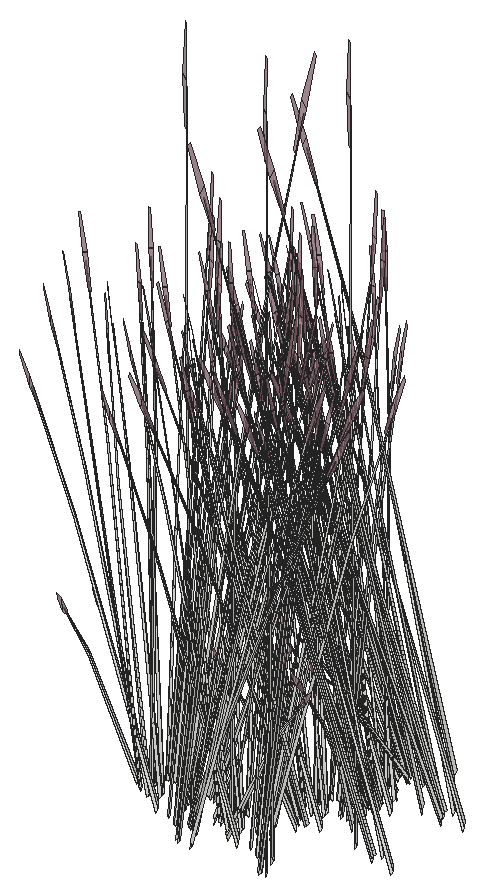
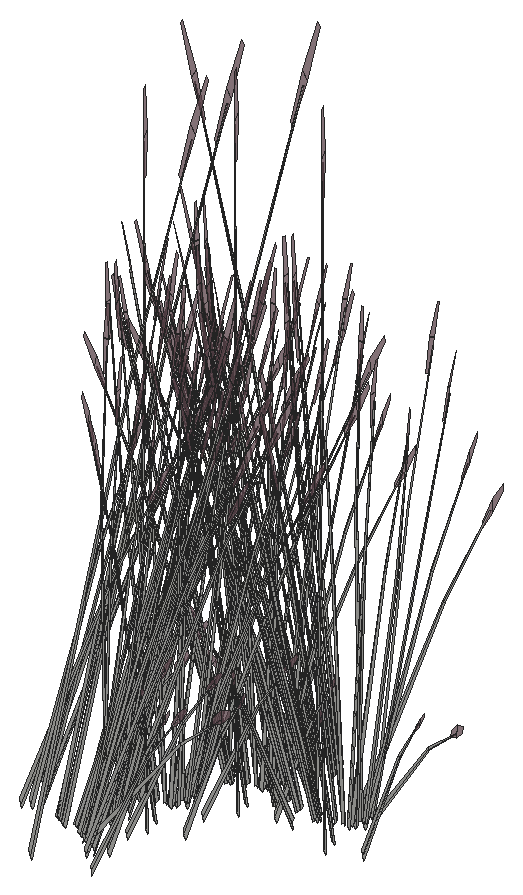
# SketchUp Ruby script. Lengths in inches.
U = 1.inch
M = Sketchup.active_model
def pt(a) = Geom::Point3d.new(a.map { |v| v * U })
def face(e, loops, mat)
  f = e.add_face(loops[0].map { |a| pt(a) })
  loops[1..].each { |l| e.add_face(l.map { |a| pt(a) }).erase! }
  f.material = f.back_material = mat if mat
  f
end
# faces: each face lists its corners as indices into pts; further lists are holes
def faces(e, pts, list, mat = nil) = list.each { |f| face(e, (f[0].is_a?(Array) ? f : [f]).map { |l| l.map { |i| pts[i] } }, mat) }
# xy, xz, yz: faces in a plane at the given z, y or x. An outline is a flat list of corners, or four numbers for a rectangle; further outlines are holes
def ring(l) = l.size == 4 ? [[l[0], l[1]], [l[2], l[1]], [l[2], l[3]], [l[0], l[3]]] : l.each_slice(2).to_a
def flat(e, list, mat, &to3) = list.each { |f| face(e, (f[0].is_a?(Array) ? f : [f]).map { |l| ring(l).map { |u, v| to3.(u, v) } }, mat) }
def xy(e, z, list, mat = nil) = flat(e, list, mat) { |x, y| [x, y, z] }
def xz(e, y, list, mat = nil) = flat(e, list, mat) { |x, z| [x, y, z] }
def yz(e, x, list, mat = nil) = flat(e, list, mat) { |y, z| [x, y, z] }
def lines(e, pts, list) = list.each { |a, b| e.add_line(pt(pts[a]), pt(pts[b])) }
# prism: a flat outline (further loops are holes) pulled along v
def prism(e, loops, v, mat = nil)
  f = face(e, loops, mat); d = Geom::Vector3d.new(v.map { |x| x * U })
  f.pushpull(f.normal.samedirection?(d) ? d.length : -d.length)
end
def box(e, o, s, mat = nil) = prism(e, [[o, [o[0] + s[0], o[1], o[2]], [o[0] + s[0], o[1] + s[1], o[2]], [o[0], o[1] + s[1], o[2]]]], [0, 0, s[2]], mat)
def at(x, y, z, deg = 0) = Geom::Transformation.translation(pt([x, y, z])) * Geom::Transformation.rotation(ORIGIN, Z_AXIS, deg.degrees)
def axes(o, x, y, z) = Geom::Transformation.new([*x, 0, *y, 0, *z, 0, *pt(o).to_a, 1])
def part(name) = M.definitions.add(name)
# library, detail: a bought-in or finely detailed component or shape, given as its bounding box
def library(name, o, s) = part(name).tap { |d| box(d.entities, o, s) }
def detail(e, o, s) = box(e.add_group.entities, o, s)
def put(e, d, t, mat = nil) = e.add_instance(d, t).tap { |i| i.material = mat if mat }
def group(e, t, mat = nil) = e.add_group.tap { |g| g.transformation = t; g.material = mat if mat }.entities
root = M.entities
M.materials.add("LightPink_Translucent").color = [144, 107, 117]
M.materials["LightPink_Translucent"].alpha = 0.75
c1 = part("blade")
p = [[2.15,0.21,22],[0,0.17,0],[0.09,0.45,0],[2.18,0.31,22],[2.29,0.31,22],[0.38,0.45,0],
  [2.48,0.24,33],[2.49,0.24,33],[2.48,0.22,33]]
faces(c1.entities,p,[[0,1,2,3],[4,5,2,3],[6,3,4,7],[8,0,3,6]])
c2 = part("seeds")
p = [[0.3,-0.1,1.38],[-0.01,-0.03,1.59],[-0.01,-0.03,0.03],[0.14,-0.07,-0.07],[0.29,-0.03,3],[0.15,0.01,3.11]]
faces(c2.entities,p,[[0,1,2,3],[1,0,4,5]],"LightPink_Translucent")
c3 = part("blade with seeds")
put(c3.entities,c1,at(0,0,0))
put(c3.entities,c2,axes([2.4,0.25,30.99],[1.5799,-0.05474,1.17369],[-0.12525,1.92788,0.29478],[-0.07173,-0.02425,1.56792]))
put(root,c3,axes([332.89,18.93,50.44],[-0.01307,-0.23234,1.01491],[0.32652,0.16572,0.74569],[-0.06422,0.11074,0.22354]))
put(root,c3,axes([326.85,20.29,51.43],[-0.20943,0.00885,1.51428],[0.13893,-0.38357,0.12244],[0.29846,0.02372,0.64734]))
put(root,c3,axes([330.16,19.82,50.95],[0.14352,-0.05653,1.56454],[0.04949,0.39467,0.12244],[-0.31087,0.05237,0.55918]))
put(root,c3,axes([327.35,18.03,52.42],[0.36145,0.26255,-0.50118],[-0.38183,0.22994,-0.3882],[-0.055,0.1334,0.95895]))
put(root,c3,axes([333.01,18.03,52.42],[0.36145,0.26255,-0.50118],[-0.38183,0.22994,-0.3882],[-0.055,0.1334,0.95895]))
put(root,c3,axes([328.43,18.29,52.14],[0.49634,0.09796,-0.45151],[-0.17013,0.33585,-0.34973],[0.04551,0.13522,0.86392]))
put(root,c3,axes([328.71,17.59,51.43],[-0.11542,-0.12546,1.51428],[0.53333,-0.10562,0.12244],[0.12054,0.19696,0.64734]))
put(root,c3,axes([331.92,23.125,51.43],[0.18755,0.06732,1.51428],[-0.38813,0.28243,0.12244],[-0.24191,-0.12741,0.64734]))
put(root,c3,axes([324.34,20.13,50.95],[0.14352,-0.05653,1.56454],[0.04949,0.39467,0.12244],[-0.31087,0.05237,0.55918]))
put(root,c3,axes([328.2,18.49,52],[-0.15222,0.30049,-0.31292],[-0.44409,-0.08764,0.40398],[0.04072,0.12098,0.77298]))
put(root,c3,axes([329.17,20.04,52.14],[-0.13679,0.35544,-0.45151],[-0.46898,-0.12183,-0.34973],[-0.18882,0.03259,0.86392]))
put(root,c3,axes([328.89,20.75,50.44],[-0.31197,0.06451,1.01491],[0.14684,-0.26661,0.74569],[0.1655,0.01824,0.22354]))
put(root,c3,axes([329.15,19.73,52.45],[0.25405,0.35383,-0.10745],[-0.45089,0.17388,-0.59638],[-0.19001,0.04668,0.90619]))
put(root,c3,axes([332.83,22.93,52.14],[-0.49824,0.09289,-0.45151],[-0.08716,-0.35177,-0.34973],[-0.13382,-0.10081,0.86392]))
put(root,c3,axes([327.24,17.91,52.72],[-0.01314,0.36145,-0.69681],[-0.55324,-0.02428,0.08409],[-0.05838,0.15313,0.9857]))
put(root,c3,axes([332.9,17.91,52.72],[-0.01314,0.36145,-0.69681],[-0.55324,-0.02428,0.08409],[-0.05838,0.15313,0.9857]))
put(root,c3,axes([338.15,22.06,52.4],[-0.50473,-0.00941,-0.62776],[0.0339,-0.39618,0.07576],[-0.21383,-0.04181,0.88802]))
put(root,c3,axes([327.76,17.66,51.43],[-0.01236,-0.14998,1.51428],[0.53562,0.09949,0.12244],[-0.03313,0.21373,0.64734]))
put(root,c3,axes([333.42,17.66,51.43],[-0.01236,-0.14998,1.51428],[0.53562,0.09949,0.12244],[-0.03313,0.21373,0.64734]))
put(root,c3,axes([322.8,20.39,52.17],[-0.08245,0.05073,1.54581],[0.00701,0.37067,-0.24447],[-0.18899,0.0482,0.12397]))
put(root,c3,axes([323.35,20.34,52.14],[-0.13679,0.35544,-0.45151],[-0.46898,-0.12183,-0.34973],[-0.18882,0.03259,0.86392]))
put(root,c3,axes([323.33,20.04,52.45],[0.25405,0.35383,-0.10745],[-0.45089,0.17388,-0.59638],[-0.19001,0.04668,0.90619]))
put(root,c3,axes([328.35,21.58,51.47],[-0.09664,-0.32847,-0.03085],[0.45676,-0.07551,-0.13989],[0.09538,0.02082,0.4614]))
put(root,c3,axes([327.16,21.57,52.45],[0.02704,-0.39739,-0.10745],[0.51189,0.01086,-0.59638],[0.19715,0.0276,0.90619]))
put(root,c3,axes([328.25,18.22,52.4],[0.24099,0.31773,-0.62776],[-0.49607,0.17707,0.07576],[0.05635,0.15352,0.88802]))
put(root,c3,axes([334.06,25.06,50.9375],[0.43633,0.15757,1.33654],[-0.42745,0.33945,0.52853],[-0.19146,-0.20119,1.12046]))
put(root,c3,axes([329.15,20.22,51.43],[0.17519,-0.08265,1.51428],[0.14749,0.38193,0.12244],[-0.27504,0.08632,0.64734]))
put(root,c3,axes([327.06,18.42,50.97],[0.01109,-0.20172,1.3638],[0.49896,0.10655,0.18846],[-0.04323,0.21498,0.64398]))
put(root,c3,axes([332.71,18.42,50.97],[0.01109,-0.20172,1.3638],[0.49896,0.10655,0.18846],[-0.04323,0.21498,0.64398]))
put(root,c3,axes([323.34,20.53,51.43],[0.17519,-0.08265,1.51428],[0.14749,0.38193,0.12244],[-0.27504,0.08632,0.64734]))
put(root,c3,axes([337.52,22.42,51.43],[0.20943,-0.00885,1.51428],[-0.13893,0.38357,0.12244],[-0.29846,-0.02372,0.64734]))
put(root,c3,axes([331.85,23.22,52],[-0.28729,-0.24465,-0.31292],[0.32804,-0.23159,0.40398],[-0.16667,-0.03524,0.77298]))
put(root,c3,axes([327.1875,21.375,52.4],[0.50473,0.00941,-0.62776],[-0.0339,0.39618,0.07576],[0.21383,0.04181,0.88802]))
put(root,c3,axes([328.24,21.56,50.44],[0.21042,-0.1771,1.01491],[0.08303,0.28036,0.74569],[-0.15207,0.0502,0.22354]))
put(root,c3,axes([329.04,20.79,52],[-0.43951,0.05584,-0.31292],[-0.11606,-0.31924,0.40398],[-0.12595,0.08575,0.77298]))
put(root,c3,axes([332.15,23.39,52.4],[-0.50473,-0.00941,-0.62776],[0.0339,-0.39618,0.07576],[-0.21383,-0.04181,0.88802]))
put(root,c3,axes([322.43,21.86,50.44],[0.21042,-0.1771,1.01491],[0.08303,0.28036,0.74569],[-0.15207,0.0502,0.22354]))
put(root,c3,axes([327.49,21.54,52],[0.28729,0.24465,-0.31292],[-0.32804,0.23159,0.40398],[0.16667,0.03524,0.77298]))
put(root,c3,axes([323.22,21.1,52],[-0.43951,0.05584,-0.31292],[-0.11606,-0.31924,0.40398],[-0.12595,0.08575,0.77298]))
put(root,c3,axes([329.17,20.57,52.45],[0.46706,0.21546,-0.10745],[-0.26908,0.31203,-0.59638],[-0.13196,0.10846,0.90619]))
put(root,c3,axes([329.8,20.48,51.43],[0.12611,-0.12006,1.51428],[0.31843,0.32408,0.12244],[-0.2184,0.14759,0.64734]))
put(root,c3,axes([337.34,22.75,52],[-0.41962,-0.10901,-0.31292],[0.12239,-0.31802,0.40398],[-0.16894,0.02916,0.77298]))
put(root,c3,axes([326.46,20.91,51.43],[-0.18755,-0.06732,1.51428],[0.38813,-0.28243,0.12244],[0.24191,0.12741,0.64734]))
put(root,c3,axes([331.98,23.47,52.14],[-0.36663,0.25884,-0.45151],[-0.32109,-0.27343,-0.34973],[-0.18628,-0.03938,0.86392]))
put(root,c3,axes([329.4,20.83,52.14],[0.12971,0.3568,-0.45151],[-0.49122,0.06241,-0.34973],[-0.14077,0.09583,0.86392]))
put(root,c3,axes([326.49,20.02,51.95],[-0.4363,-0.20303,1.22187],[0.46069,-0.31611,0.5272],[0.14077,0.1905,1.18105]))
put(root,c3,axes([334.54,26.51,51.43],[0.11542,0.12546,1.51428],[-0.53333,0.10562,0.12244],[-0.12054,-0.19696,0.64734]))
put(root,c3,axes([331.16,23.81,50.44],[0.32236,-0.02796,1.01491],[-0.20448,0.24636,0.74569],[-0.1593,-0.03696,0.22354]))
put(root,c3,axes([323.35,20.88,52.45],[0.46706,0.21546,-0.10745],[-0.26908,0.31203,-0.59638],[-0.13196,0.10846,0.90619]))
put(root,c3,axes([332.28,20.1,50.51],[-0.01379,-0.36791,1.24828],[0.62424,0.09537,0.52853],[-0.14764,0.20132,1.17828]))
put(root,c3,axes([327.15,21.68,50.44],[-0.28429,-0.11236,1.01491],[0.36709,-0.11416,0.74569],[0.09901,0.0967,0.22354]))
put(root,c3,axes([332.18,23.19,52.45],[-0.02704,0.39739,-0.10745],[-0.51189,-0.01086,-0.59638],[-0.19715,-0.0276,0.90619]))
put(root,c3,axes([326.15,22,52.45],[0.30087,-0.33447,-0.10745],[0.43572,0.19269,-0.59638],[0.15146,0.0945,0.90619]))
put(root,c3,axes([323.98,20.78,51.43],[0.12611,-0.12006,1.51428],[0.31843,0.32408,0.12244],[-0.2184,0.14759,0.64734]))
put(root,c3,axes([331.52,23.74,51.43],[0.20943,-0.00885,1.51428],[-0.13893,0.38357,0.12244],[-0.29846,-0.02372,0.64734]))
put(root,c3,axes([323.58,21.14,52.14],[0.12971,0.3568,-0.45151],[-0.49122,0.06241,-0.34973],[-0.14077,0.09583,0.86392]))
put(root,c3,axes([326.46,20.41,50.51],[-0.01379,-0.36791,1.24828],[0.62424,0.09537,0.52853],[-0.14764,0.20132,1.17828]))
put(root,c3,axes([326.51,21.83,52.14],[0.49824,-0.09289,-0.45151],[0.08716,0.35177,-0.34973],[0.13382,0.10081,0.86392]))
put(root,c3,axes([338.62,22.69,50.95],[0.14352,-0.05653,1.56454],[0.04949,0.39467,0.12244],[-0.31087,0.05237,0.55918]))
put(root,c3,axes([329.7,20.77,51.43],[0.09401,-0.13431,1.51428],[0.3944,0.27795,0.12244],[-0.17792,0.17323,0.64734]))
put(root,c3,axes([329.81,21.53,52],[-0.34164,0.20573,-0.31292],[-0.3234,-0.23491,0.40398],[-0.04921,0.11936,0.77298]))
put(root,c3,axes([330.8,21.7,52.45],[0.49409,-0.18193,-0.10745],[0.24281,0.32289,-0.59638],[0.06519,0.13607,0.90619]))
put(root,c3,axes([330.03,22.33,50.44],[-0.01307,-0.23234,1.01491],[0.32652,0.16572,0.74569],[-0.06422,0.11074,0.22354]))
put(root,c3,axes([323.88,21.08,51.43],[0.09401,-0.13431,1.51428],[0.3944,0.27795,0.12244],[-0.17792,0.17323,0.64734]))
put(root,c3,axes([323.99,21.84,52],[-0.34164,0.20573,-0.31292],[-0.3234,-0.23491,0.40398],[-0.04921,0.11936,0.77298]))
put(root,c3,axes([330.15,21.43,52.42],[0.36145,0.26255,-0.50118],[-0.38183,0.22994,-0.3882],[-0.055,0.1334,0.95895]))
put(root,c3,axes([324.98,22.01,52.45],[0.49409,-0.18193,-0.10745],[0.24281,0.32289,-0.59638],[0.06519,0.13607,0.90619]))
put(root,c3,axes([334.24,25.97,50.44],[0.26338,0.136,1.01491],[-0.38358,0.08175,0.74569],[-0.08207,-0.10452,0.22354]))
put(root,c3,axes([334.87,26.69,52.4],[-0.43054,-0.18887,-0.62776],[0.30598,-0.33097,0.07576],[-0.15599,-0.11277,0.88802]))
put(root,c3,axes([334.72,26.44,52],[-0.07798,-0.31474,-0.31292],[0.44579,-0.08311,0.40398],[-0.11974,-0.09019,0.77298]))
put(root,c3,axes([324.21,22.64,50.44],[-0.01307,-0.23234,1.01491],[0.32652,0.16572,0.74569],[-0.06422,0.11074,0.22354]))
put(root,c3,axes([331.22,21.6875,52.14],[0.49634,0.09796,-0.45151],[-0.17013,0.33585,-0.34973],[0.04551,0.13522,0.86392]))
put(root,c3,axes([331.5,20.99,51.43],[-0.11542,-0.12546,1.51428],[0.53333,-0.10562,0.12244],[0.12054,0.19696,0.64734]))
put(root,c3,axes([331.34,24.07,52],[-0.41962,-0.10901,-0.31292],[0.12239,-0.31802,0.40398],[-0.16894,0.02916,0.77298]))
put(root,c3,axes([331,21.89,52],[-0.15222,0.30049,-0.31292],[-0.44409,-0.08764,0.40398],[0.04072,0.12098,0.77298]))
put(root,c3,axes([324.33,21.74,52.42],[0.36145,0.26255,-0.50118],[-0.38183,0.22994,-0.3882],[-0.055,0.1334,0.95895]))
put(root,c3,axes([330.04,21.3125,52.72],[-0.01314,0.36145,-0.69681],[-0.55324,-0.02428,0.08409],[-0.05838,0.15313,0.9857]))
put(root,c3,axes([337.61,23.09,51.43],[0.17519,-0.08265,1.51428],[0.14749,0.38193,0.12244],[-0.27504,0.08632,0.64734]))
put(root,c3,axes([325.4,22,52.14],[0.49634,0.09796,-0.45151],[-0.17013,0.33585,-0.34973],[0.04551,0.13522,0.86392]))
put(root,c3,axes([325.6875,21.3,51.43],[-0.11542,-0.12546,1.51428],[0.53333,-0.10562,0.12244],[0.12054,0.19696,0.64734]))
put(root,c3,axes([330.5625,21.06,51.43],[-0.01236,-0.14998,1.51428],[0.53562,0.09949,0.12244],[-0.03313,0.21373,0.64734]))
put(root,c3,axes([333.76,26.9,51.43],[0.18755,0.06732,1.51428],[-0.38813,0.28243,0.12244],[-0.24191,-0.12741,0.64734]))
put(root,c3,axes([325.18,22.2,52],[-0.15222,0.30049,-0.31292],[-0.44409,-0.08764,0.40398],[0.04072,0.12098,0.77298]))
put(root,c3,axes([331.04,21.625,52.4],[0.24099,0.31773,-0.62776],[-0.49607,0.17707,0.07576],[0.05635,0.15352,0.88802]))
put(root,c3,axes([324.22,21.62,52.72],[-0.01314,0.36145,-0.69681],[-0.55324,-0.02428,0.08409],[-0.05838,0.15313,0.9857]))
put(root,c3,axes([334.67,26.7,52.14],[-0.49824,0.09289,-0.45151],[-0.08716,-0.35177,-0.34973],[-0.13382,-0.10081,0.86392]))
put(root,c3,axes([332.62,24.02,50.95],[0.14352,-0.05653,1.56454],[0.04949,0.39467,0.12244],[-0.31087,0.05237,0.55918]))
put(root,c3,axes([324.74,21.36,51.43],[-0.01236,-0.14998,1.51428],[0.53562,0.09949,0.12244],[-0.03313,0.21373,0.64734]))
put(root,c3,axes([325.22,21.93,52.4],[0.24099,0.31773,-0.62776],[-0.49607,0.17707,0.07576],[0.05635,0.15352,0.88802]))
put(root,c3,axes([331.63,24.23,52.14],[-0.13679,0.35544,-0.45151],[-0.46898,-0.12183,-0.34973],[-0.18882,0.03259,0.86392]))
put(root,c3,axes([331.61,23.93,52.45],[0.25405,0.35383,-0.10745],[-0.45089,0.17388,-0.59638],[-0.19001,0.04668,0.90619]))
put(root,c3,axes([329.85,21.82,50.97],[0.01109,-0.20172,1.3638],[0.49896,0.10655,0.18846],[-0.04323,0.21498,0.64398]))
put(root,c3,axes([335.9,28.83,50.9375],[0.43633,0.15757,1.33654],[-0.42745,0.33945,0.52853],[-0.19146,-0.20119,1.12046]))
put(root,c3,axes([324.04,22.13,50.97],[0.01109,-0.20172,1.3638],[0.49896,0.10655,0.18846],[-0.04323,0.21498,0.64398]))
put(root,c3,axes([337.92,27.99,51.43],[0.18755,0.06732,1.51428],[-0.38813,0.28243,0.12244],[-0.24191,-0.12741,0.64734]))
put(root,c3,axes([331.61,24.42,51.43],[0.17519,-0.08265,1.51428],[0.14749,0.38193,0.12244],[-0.27504,0.08632,0.64734]))
put(root,c3,axes([333.69,26.99,52],[-0.28729,-0.24465,-0.31292],[0.32804,-0.23159,0.40398],[-0.16667,-0.03524,0.77298]))
put(root,c3,axes([333.99,27.16,52.4],[-0.50473,-0.00941,-0.62776],[0.0339,-0.39618,0.07576],[-0.21383,-0.04181,0.88802]))
put(root,c3,axes([330.7,25.75,50.44],[0.21042,-0.1771,1.01491],[0.08303,0.28036,0.74569],[-0.15207,0.0502,0.22354]))
put(root,c3,axes([331.49,24.99,52],[-0.43951,0.05584,-0.31292],[-0.11606,-0.31924,0.40398],[-0.12595,0.08575,0.77298]))
put(root,c3,axes([333.83,27.24,52.14],[-0.36663,0.25884,-0.45151],[-0.32109,-0.27343,-0.34973],[-0.18628,-0.03938,0.86392]))
put(root,c3,axes([333,27.58,50.44],[0.32236,-0.02796,1.01491],[-0.20448,0.24636,0.74569],[-0.1593,-0.03696,0.22354]))
put(root,c3,axes([334.02,26.97,52.45],[-0.02704,0.39739,-0.10745],[-0.51189,-0.01086,-0.59638],[-0.19715,-0.0276,0.90619]))
put(root,c3,axes([331.625,24.77,52.45],[0.46706,0.21546,-0.10745],[-0.26908,0.31203,-0.59638],[-0.13196,0.10846,0.90619]))
put(root,c3,axes([333.63,30.48,51.43],[0.11542,0.12546,1.51428],[-0.53333,0.10562,0.12244],[-0.12054,-0.19696,0.64734]))
put(root,c3,axes([333.37,27.51,51.43],[0.20943,-0.00885,1.51428],[-0.13893,0.38357,0.12244],[-0.29846,-0.02372,0.64734]))
put(root,c3,axes([334.51,29.65,52.17],[-0.07723,-0.05479,1.54581],[-0.51538,0.03473,-0.24447],[-0.08225,-0.13104,0.12397]))
put(root,c3,axes([332.25,24.67,51.43],[0.12611,-0.12006,1.51428],[0.31843,0.32408,0.12244],[-0.2184,0.14759,0.64734]))
put(root,c3,axes([331.86,25.03,52.14],[0.12971,0.3568,-0.45151],[-0.49122,0.06241,-0.34973],[-0.14077,0.09583,0.86392]))
put(root,c3,axes([335.05,30.57,52.4],[-0.24099,-0.31773,-0.62776],[0.49607,-0.17707,0.07576],[-0.05635,-0.15352,0.88802]))
put(root,c3,axes([338.15,28.25,52.4],[-0.50473,-0.00941,-0.62776],[0.0339,-0.39618,0.07576],[-0.21383,-0.04181,0.88802]))
put(root,c3,axes([334.74,24.3,50.51],[-0.01379,-0.36791,1.24828],[0.62424,0.09537,0.52853],[-0.14764,0.20132,1.17828]))
put(root,c3,axes([334.87,30.51,52.14],[-0.49634,-0.09796,-0.45151],[0.17013,-0.33585,-0.34973],[-0.04551,-0.13522,0.86392]))
put(root,c3,axes([332.16,24.97,51.43],[0.09401,-0.13431,1.51428],[0.3944,0.27795,0.12244],[-0.17792,0.17323,0.64734]))
put(root,c3,axes([332.27,25.73,52],[-0.34164,0.20573,-0.31292],[-0.3234,-0.23491,0.40398],[-0.04921,0.11936,0.77298]))
put(root,c3,axes([333.18,27.84,52],[-0.41962,-0.10901,-0.31292],[0.12239,-0.31802,0.40398],[-0.16894,0.02916,0.77298]))
put(root,c3,axes([335.29,30.49,52.45],[-0.49409,0.18193,-0.10745],[-0.24281,-0.32289,-0.59638],[-0.06519,-0.13607,0.90619]))
put(root,c3,axes([332.48,26.53,50.44],[-0.01307,-0.23234,1.01491],[0.32652,0.16572,0.74569],[-0.06422,0.11074,0.22354]))
put(root,c3,axes([337.52,28.61,51.43],[0.20943,-0.00885,1.51428],[-0.13893,0.38357,0.12244],[-0.29846,-0.02372,0.64734]))
put(root,c3,axes([333.33,29.94,50.44],[0.26338,0.136,1.01491],[-0.38358,0.08175,0.74569],[-0.08207,-0.10452,0.22354]))
put(root,c3,axes([333.96,30.66,52.4],[-0.43054,-0.18887,-0.62776],[0.30598,-0.33097,0.07576],[-0.15599,-0.11277,0.88802]))
put(root,c3,axes([333.8125,30.41,52],[-0.07798,-0.31474,-0.31292],[0.44579,-0.08311,0.40398],[-0.11974,-0.09019,0.77298]))
put(root,c3,axes([332.61,25.63,52.42],[0.36145,0.26255,-0.50118],[-0.38183,0.22994,-0.3882],[-0.055,0.1334,0.95895]))
put(root,c3,axes([332.85,30.87,51.43],[0.18755,0.06732,1.51428],[-0.38813,0.28243,0.12244],[-0.24191,-0.12741,0.64734]))
put(root,c3,axes([334.46,27.79,50.95],[0.14352,-0.05653,1.56454],[0.04949,0.39467,0.12244],[-0.31087,0.05237,0.55918]))
put(root,c3,axes([332.49,25.51,52.72],[-0.01314,0.36145,-0.69681],[-0.55324,-0.02428,0.08409],[-0.05838,0.15313,0.9857]))
put(root,c3,axes([333.76,30.67,52.14],[-0.49824,0.09289,-0.45151],[-0.08716,-0.35177,-0.34973],[-0.13382,-0.10081,0.86392]))
put(root,c3,axes([333.02,25.25,51.43],[-0.01236,-0.14998,1.51428],[0.53562,0.09949,0.12244],[-0.03313,0.21373,0.64734]))
put(root,c3,axes([333.47,28.01,52.14],[-0.13679,0.35544,-0.45151],[-0.46898,-0.12183,-0.34973],[-0.18882,0.03259,0.86392]))
put(root,c3,axes([333.45,27.7,52.45],[0.25405,0.35383,-0.10745],[-0.45089,0.17388,-0.59638],[-0.19001,0.04668,0.90619]))
put(root,c3,axes([337.34,28.9375,52],[-0.41962,-0.10901,-0.31292],[0.12239,-0.31802,0.40398],[-0.16894,0.02916,0.77298]))
put(root,c3,axes([332.82,30.25,52.17],[-0.10864,-0.00276,1.54581],[-0.34587,0.27582,-0.24447],[-0.18454,-0.05636,0.12397]))
put(root,c3,axes([334.99,32.8,50.9375],[0.43633,0.15757,1.33654],[-0.42745,0.33945,0.52853],[-0.19146,-0.20119,1.12046]))
put(root,c3,axes([332.31,26.02,50.97],[0.01109,-0.20172,1.3638],[0.49896,0.10655,0.18846],[-0.04323,0.21498,0.64398]))
put(root,c3,axes([333.46,28.1875,51.43],[0.17519,-0.08265,1.51428],[0.14749,0.38193,0.12244],[-0.27504,0.08632,0.64734]))
put(root,c3,axes([338.62,28.88,50.95],[0.14352,-0.05653,1.56454],[0.04949,0.39467,0.12244],[-0.31087,0.05237,0.55918]))
put(root,c3,axes([332.78,30.97,52],[-0.28729,-0.24465,-0.31292],[0.32804,-0.23159,0.40398],[-0.16667,-0.03524,0.77298]))
put(root,c3,axes([332.54,29.53,50.44],[0.21042,-0.1771,1.01491],[0.08303,0.28036,0.74569],[-0.15207,0.0502,0.22354]))
put(root,c3,axes([333.09,31.13,52.4],[-0.50473,-0.00941,-0.62776],[0.0339,-0.39618,0.07576],[-0.21383,-0.04181,0.88802]))
put(root,c3,axes([333.34,28.76,52],[-0.43951,0.05584,-0.31292],[-0.11606,-0.31924,0.40398],[-0.12595,0.08575,0.77298]))
put(root,c3,axes([337.61,29.28,51.43],[0.17519,-0.08265,1.51428],[0.14749,0.38193,0.12244],[-0.27504,0.08632,0.64734]))
put(root,c3,axes([332.92,31.21,52.14],[-0.36663,0.25884,-0.45151],[-0.32109,-0.27343,-0.34973],[-0.18628,-0.03938,0.86392]))
put(root,c3,axes([333.47,28.54,52.45],[0.46706,0.21546,-0.10745],[-0.26908,0.31203,-0.59638],[-0.13196,0.10846,0.90619]))
put(root,c3,axes([332.09,31.55,50.44],[0.32236,-0.02796,1.01491],[-0.20448,0.24636,0.74569],[-0.1593,-0.03696,0.22354]))
put(root,c3,axes([333.11,30.9375,52.45],[-0.02704,0.39739,-0.10745],[-0.51189,-0.01086,-0.59638],[-0.19715,-0.0276,0.90619]))
put(root,c3,axes([334.1,28.45,51.43],[0.12611,-0.12006,1.51428],[0.31843,0.32408,0.12244],[-0.2184,0.14759,0.64734]))
put(root,c3,axes([333.7,28.8,52.14],[0.12971,0.3568,-0.45151],[-0.49122,0.06241,-0.34973],[-0.14077,0.09583,0.86392]))
put(root,c3,axes([332.46,31.49,51.43],[0.20943,-0.00885,1.51428],[-0.13893,0.38357,0.12244],[-0.29846,-0.02372,0.64734]))
